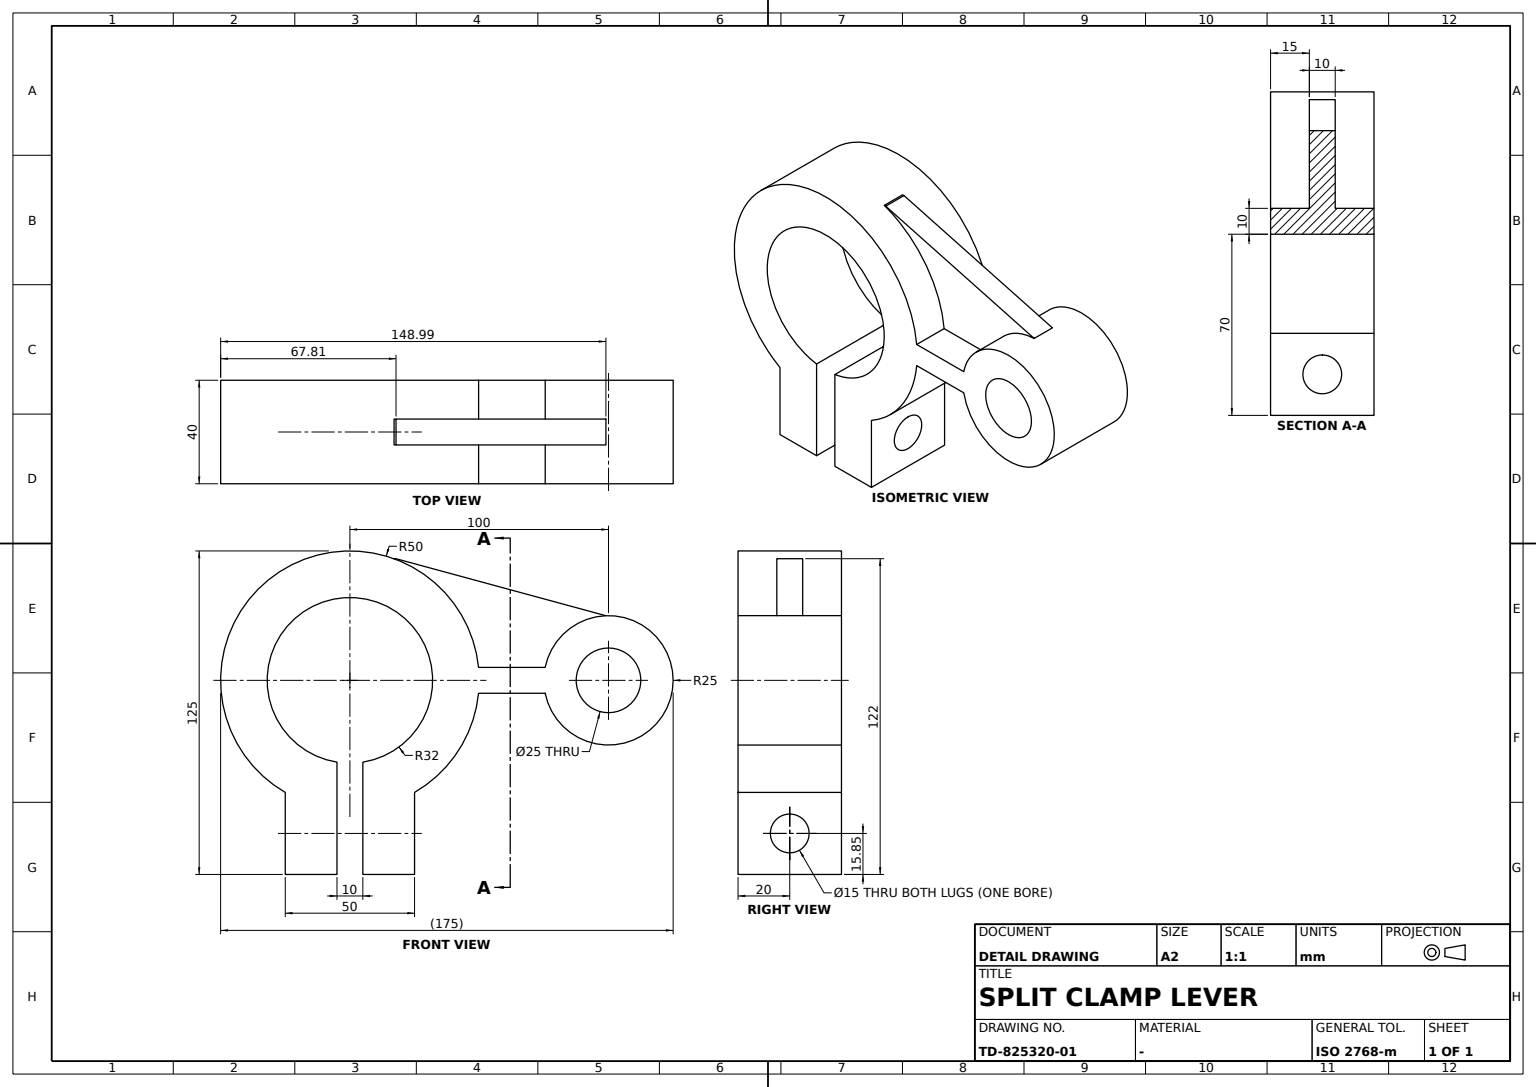
ISO-10303-21;
HEADER;
FILE_DESCRIPTION((''),'2;1');
FILE_NAME('','',(''),(''),'','','');
FILE_SCHEMA(('AUTOMOTIVE_DESIGN'));
ENDSEC;
DATA;
#1=APPLICATION_CONTEXT('');
#2=PRODUCT_CONTEXT('',#1,'mechanical');
#3=PRODUCT('','','',(#2));
#4=PRODUCT_DEFINITION_FORMATION('','',#3);
#5=PRODUCT_DEFINITION_CONTEXT('',#1,'design');
#6=PRODUCT_DEFINITION('','',#4,#5);
#7=PRODUCT_DEFINITION_SHAPE('','',#6);
#8=(LENGTH_UNIT()NAMED_UNIT(*)SI_UNIT(.MILLI.,.METRE.));
#9=(NAMED_UNIT(*)PLANE_ANGLE_UNIT()SI_UNIT($,.RADIAN.));
#10=(NAMED_UNIT(*)SI_UNIT($,.STERADIAN.)SOLID_ANGLE_UNIT());
#11=UNCERTAINTY_MEASURE_WITH_UNIT(LENGTH_MEASURE(0.005),#8,'distance_accuracy_value','');
#12=(GEOMETRIC_REPRESENTATION_CONTEXT(3)GLOBAL_UNCERTAINTY_ASSIGNED_CONTEXT((#11))GLOBAL_UNIT_ASSIGNED_CONTEXT((#8,#9,#10))REPRESENTATION_CONTEXT('',''));
#13=CARTESIAN_POINT('',(5.,116.108107,99.979388));
#14=VERTEX_POINT('',#13);
#15=CARTESIAN_POINT('',(5.,34.936643,122.));
#16=VERTEX_POINT('',#15);
#17=DIRECTION('',(0.,-0.965116262,0.261821696));
#18=VECTOR('',#17,1000.);
#19=LINE('',#13,#18);
#20=EDGE_CURVE('',#14,#16,#19,.T.);
#21=ORIENTED_EDGE('',*,*,#20,.T.);
#22=CARTESIAN_POINT('',(5.,34.181796,122.));
#23=VERTEX_POINT('',#22);
#24=CARTESIAN_POINT('',(5.,129.288452,122.));
#25=DIRECTION('',(0.,-1.,0.));
#26=VECTOR('',#25,1000.);
#27=LINE('',#24,#26);
#28=EDGE_CURVE('',#16,#23,#27,.T.);
#29=ORIENTED_EDGE('',*,*,#28,.T.);
#30=CARTESIAN_POINT('',(5.,66.872445,80.));
#31=VERTEX_POINT('',#30);
#32=CARTESIAN_POINT('',(5.,17.123074,75.));
#33=DIRECTION('',(1.,0.,0.));
#34=DIRECTION('',(0.,0.,-1.));
#35=AXIS2_PLACEMENT_3D('',#32,#33,#34);
#36=CIRCLE('',#35,50.);
#37=EDGE_CURVE('',#31,#23,#36,.T.);
#38=ORIENTED_EDGE('',*,*,#37,.F.);
#39=CARTESIAN_POINT('',(5.,92.628176,80.));
#40=VERTEX_POINT('',#39);
#41=CARTESIAN_POINT('',(5.,129.288452,80.));
#42=DIRECTION('',(0.,1.,0.));
#43=VECTOR('',#42,1000.);
#44=LINE('',#41,#43);
#45=EDGE_CURVE('',#31,#40,#44,.T.);
#46=ORIENTED_EDGE('',*,*,#45,.T.);
#47=CARTESIAN_POINT('',(5.,117.123074,75.));
#48=AXIS2_PLACEMENT_3D('',#47,#33,#34);
#49=CIRCLE('',#48,25.);
#50=EDGE_CURVE('',#14,#40,#49,.T.);
#51=ORIENTED_EDGE('',*,*,#50,.F.);
#52=EDGE_LOOP('',(#21,#29,#38,#46,#51));
#53=FACE_BOUND('',#52,.T.);
#54=CARTESIAN_POINT('',(5.,129.288452,114.));
#55=AXIS2_PLACEMENT_3D('',#54,#33,#25);
#56=PLANE('',#55);
#57=ADVANCED_FACE('',(#53),#56,.T.);
#58=CARTESIAN_POINT('',(-5.,34.181796,122.));
#59=VERTEX_POINT('',#58);
#60=VECTOR('',#33,1000.);
#61=LINE('',#22,#60);
#62=EDGE_CURVE('',#23,#59,#61,.F.);
#63=ORIENTED_EDGE('',*,*,#62,.F.);
#64=ORIENTED_EDGE('',*,*,#28,.F.);
#65=CARTESIAN_POINT('',(-5.,34.936643,122.));
#66=VERTEX_POINT('',#65);
#67=DIRECTION('',(-1.,0.,0.));
#68=VECTOR('',#67,1000.);
#69=LINE('',#15,#68);
#70=EDGE_CURVE('',#16,#66,#69,.T.);
#71=ORIENTED_EDGE('',*,*,#70,.T.);
#72=CARTESIAN_POINT('',(-5.,19.127685,122.));
#73=LINE('',#72,#43);
#74=EDGE_CURVE('',#59,#66,#73,.T.);
#75=ORIENTED_EDGE('',*,*,#74,.F.);
#76=EDGE_LOOP('',(#63,#64,#71,#75));
#77=FACE_BOUND('',#76,.T.);
#78=CARTESIAN_POINT('',(0.,0.,122.));
#79=DIRECTION('',(0.,0.,1.));
#80=AXIS2_PLACEMENT_3D('',#78,#79,#67);
#81=PLANE('',#80);
#82=ADVANCED_FACE('',(#77),#81,.T.);
#83=CARTESIAN_POINT('',(0.,12.123074,8.3495));
#84=VERTEX_POINT('',#83);
#85=CARTESIAN_POINT('',(0.,12.123074,15.8495));
#86=AXIS2_PLACEMENT_3D('',#85,#25,#34);
#87=CIRCLE('',#86,7.5);
#88=EDGE_CURVE('',#84,#84,#87,.T.);
#89=ORIENTED_EDGE('',*,*,#88,.F.);
#90=EDGE_LOOP('',(#89));
#91=FACE_BOUND('',#90,.T.);
#92=CARTESIAN_POINT('',(0.,-7.876926,8.3495));
#93=VERTEX_POINT('',#92);
#94=CARTESIAN_POINT('',(0.,-7.876926,15.8495));
#95=AXIS2_PLACEMENT_3D('',#94,#25,#34);
#96=CIRCLE('',#95,7.5);
#97=EDGE_CURVE('',#93,#93,#96,.T.);
#98=ORIENTED_EDGE('',*,*,#97,.T.);
#99=EDGE_LOOP('',(#98));
#100=FACE_BOUND('',#99,.T.);
#101=CARTESIAN_POINT('',(0.,42.023074,15.8495));
#102=AXIS2_PLACEMENT_3D('',#101,#25,#33);
#103=CYLINDRICAL_SURFACE('',#102,7.5);
#104=ADVANCED_FACE('',(#91,#100),#103,.F.);
#105=CARTESIAN_POINT('',(-20.,22.123074,0.));
#106=VERTEX_POINT('',#105);
#107=CARTESIAN_POINT('',(20.,22.123074,0.));
#108=VERTEX_POINT('',#107);
#109=CARTESIAN_POINT('',(0.,22.123074,0.));
#110=LINE('',#109,#60);
#111=EDGE_CURVE('',#106,#108,#110,.T.);
#112=ORIENTED_EDGE('',*,*,#111,.F.);
#113=CARTESIAN_POINT('',(-20.,42.123074,0.));
#114=VERTEX_POINT('',#113);
#115=CARTESIAN_POINT('',(-20.,0.,0.));
#116=LINE('',#115,#26);
#117=EDGE_CURVE('',#114,#106,#116,.T.);
#118=ORIENTED_EDGE('',*,*,#117,.F.);
#119=CARTESIAN_POINT('',(20.,42.123074,0.));
#120=VERTEX_POINT('',#119);
#121=CARTESIAN_POINT('',(0.,42.123074,0.));
#122=LINE('',#121,#60);
#123=EDGE_CURVE('',#114,#120,#122,.T.);
#124=ORIENTED_EDGE('',*,*,#123,.T.);
#125=CARTESIAN_POINT('',(20.,0.,0.));
#126=LINE('',#125,#26);
#127=EDGE_CURVE('',#120,#108,#126,.T.);
#128=ORIENTED_EDGE('',*,*,#127,.T.);
#129=EDGE_LOOP('',(#112,#118,#124,#128));
#130=FACE_BOUND('',#129,.T.);
#131=CARTESIAN_POINT('',(0.,12.123074,0.));
#132=AXIS2_PLACEMENT_3D('',#131,#79,#25);
#133=PLANE('',#132);
#134=ADVANCED_FACE('',(#130),#133,.F.);
#135=CARTESIAN_POINT('',(-20.,66.872445,80.));
#136=VERTEX_POINT('',#135);
#137=CARTESIAN_POINT('',(-5.,66.872445,80.));
#138=VERTEX_POINT('',#137);
#139=LINE('',#135,#60);
#140=EDGE_CURVE('',#136,#138,#139,.T.);
#141=ORIENTED_EDGE('',*,*,#140,.T.);
#142=CARTESIAN_POINT('',(-5.,92.628176,80.));
#143=VERTEX_POINT('',#142);
#144=LINE('',#137,#43);
#145=EDGE_CURVE('',#138,#143,#144,.T.);
#146=ORIENTED_EDGE('',*,*,#145,.T.);
#147=CARTESIAN_POINT('',(-20.,92.628176,80.));
#148=VERTEX_POINT('',#147);
#149=LINE('',#147,#60);
#150=EDGE_CURVE('',#148,#143,#149,.T.);
#151=ORIENTED_EDGE('',*,*,#150,.F.);
#152=CARTESIAN_POINT('',(-20.,0.,80.));
#153=LINE('',#152,#43);
#154=EDGE_CURVE('',#136,#148,#153,.T.);
#155=ORIENTED_EDGE('',*,*,#154,.F.);
#156=EDGE_LOOP('',(#141,#146,#151,#155));
#157=FACE_BOUND('',#156,.T.);
#158=CARTESIAN_POINT('',(0.,66.872445,80.));
#159=AXIS2_PLACEMENT_3D('',#158,#34,#42);
#160=PLANE('',#159);
#161=ADVANCED_FACE('',(#157),#160,.F.);
#162=CARTESIAN_POINT('',(0.,22.123074,8.3495));
#163=VERTEX_POINT('',#162);
#164=CARTESIAN_POINT('',(0.,22.123074,15.8495));
#165=AXIS2_PLACEMENT_3D('',#164,#25,#34);
#166=CIRCLE('',#165,7.5);
#167=EDGE_CURVE('',#163,#163,#166,.T.);
#168=ORIENTED_EDGE('',*,*,#167,.F.);
#169=EDGE_LOOP('',(#168));
#170=FACE_BOUND('',#169,.T.);
#171=CARTESIAN_POINT('',(-20.,22.123074,43.393039));
#172=VERTEX_POINT('',#171);
#173=VECTOR('',#34,1000.);
#174=LINE('',#105,#173);
#175=EDGE_CURVE('',#172,#106,#174,.T.);
#176=ORIENTED_EDGE('',*,*,#175,.T.);
#177=ORIENTED_EDGE('',*,*,#111,.T.);
#178=CARTESIAN_POINT('',(20.,22.123074,43.393039));
#179=VERTEX_POINT('',#178);
#180=LINE('',#107,#173);
#181=EDGE_CURVE('',#179,#108,#180,.T.);
#182=ORIENTED_EDGE('',*,*,#181,.F.);
#183=LINE('',#171,#60);
#184=EDGE_CURVE('',#172,#179,#183,.T.);
#185=ORIENTED_EDGE('',*,*,#184,.F.);
#186=EDGE_LOOP('',(#176,#177,#182,#185));
#187=FACE_BOUND('',#186,.T.);
#188=CARTESIAN_POINT('',(0.,22.123074,43.393039));
#189=AXIS2_PLACEMENT_3D('',#188,#25,#34);
#190=PLANE('',#189);
#191=ADVANCED_FACE('',(#170,#187),#190,.T.);
#192=CARTESIAN_POINT('',(20.,42.123074,31.69873));
#193=VERTEX_POINT('',#192);
#194=CARTESIAN_POINT('',(20.,66.872445,70.));
#195=VERTEX_POINT('',#194);
#196=CARTESIAN_POINT('',(20.,17.123074,75.));
#197=AXIS2_PLACEMENT_3D('',#196,#33,#34);
#198=CIRCLE('',#197,50.);
#199=EDGE_CURVE('',#193,#195,#198,.T.);
#200=ORIENTED_EDGE('',*,*,#199,.F.);
#201=CARTESIAN_POINT('',(-20.,42.123074,31.69873));
#202=VERTEX_POINT('',#201);
#203=LINE('',#201,#60);
#204=EDGE_CURVE('',#202,#193,#203,.T.);
#205=ORIENTED_EDGE('',*,*,#204,.F.);
#206=CARTESIAN_POINT('',(-20.,66.872445,70.));
#207=VERTEX_POINT('',#206);
#208=CARTESIAN_POINT('',(-20.,17.123074,75.));
#209=AXIS2_PLACEMENT_3D('',#208,#33,#34);
#210=CIRCLE('',#209,50.);
#211=EDGE_CURVE('',#202,#207,#210,.T.);
#212=ORIENTED_EDGE('',*,*,#211,.T.);
#213=LINE('',#206,#60);
#214=EDGE_CURVE('',#207,#195,#213,.T.);
#215=ORIENTED_EDGE('',*,*,#214,.T.);
#216=EDGE_LOOP('',(#200,#205,#212,#215));
#217=FACE_BOUND('',#216,.T.);
#218=CARTESIAN_POINT('',(0.,17.123074,75.));
#219=AXIS2_PLACEMENT_3D('',#218,#33,#42);
#220=CYLINDRICAL_SURFACE('',#219,50.);
#221=ADVANCED_FACE('',(#217),#220,.T.);
#222=ORIENTED_EDGE('',*,*,#97,.F.);
#223=EDGE_LOOP('',(#222));
#224=FACE_BOUND('',#223,.T.);
#225=CARTESIAN_POINT('',(-20.,-7.876926,0.));
#226=VERTEX_POINT('',#225);
#227=CARTESIAN_POINT('',(20.,-7.876926,0.));
#228=VERTEX_POINT('',#227);
#229=CARTESIAN_POINT('',(0.,-7.876926,0.));
#230=LINE('',#229,#60);
#231=EDGE_CURVE('',#226,#228,#230,.T.);
#232=ORIENTED_EDGE('',*,*,#231,.T.);
#233=CARTESIAN_POINT('',(20.,-7.876926,31.69873));
#234=VERTEX_POINT('',#233);
#235=LINE('',#227,#173);
#236=EDGE_CURVE('',#234,#228,#235,.T.);
#237=ORIENTED_EDGE('',*,*,#236,.F.);
#238=CARTESIAN_POINT('',(-20.,-7.876926,31.69873));
#239=VERTEX_POINT('',#238);
#240=LINE('',#238,#60);
#241=EDGE_CURVE('',#239,#234,#240,.T.);
#242=ORIENTED_EDGE('',*,*,#241,.F.);
#243=LINE('',#225,#173);
#244=EDGE_CURVE('',#239,#226,#243,.T.);
#245=ORIENTED_EDGE('',*,*,#244,.T.);
#246=EDGE_LOOP('',(#232,#237,#242,#245));
#247=FACE_BOUND('',#246,.T.);
#248=CARTESIAN_POINT('',(0.,-7.876926,31.69873));
#249=AXIS2_PLACEMENT_3D('',#248,#25,#34);
#250=PLANE('',#249);
#251=ADVANCED_FACE('',(#224,#247),#250,.T.);
#252=ORIENTED_EDGE('',*,*,#167,.T.);
#253=EDGE_LOOP('',(#252));
#254=FACE_BOUND('',#253,.T.);
#255=CARTESIAN_POINT('',(0.,42.123074,23.3495));
#256=VERTEX_POINT('',#255);
#257=CARTESIAN_POINT('',(0.,42.123074,15.8495));
#258=AXIS2_PLACEMENT_3D('',#257,#42,#79);
#259=CIRCLE('',#258,7.5);
#260=EDGE_CURVE('',#256,#256,#259,.T.);
#261=ORIENTED_EDGE('',*,*,#260,.T.);
#262=EDGE_LOOP('',(#261));
#263=FACE_BOUND('',#262,.T.);
#264=ADVANCED_FACE('',(#254,#263),#103,.F.);
#265=CARTESIAN_POINT('',(-20.,12.123074,0.));
#266=VERTEX_POINT('',#265);
#267=CARTESIAN_POINT('',(20.,12.123074,0.));
#268=VERTEX_POINT('',#267);
#269=LINE('',#131,#60);
#270=EDGE_CURVE('',#266,#268,#269,.T.);
#271=ORIENTED_EDGE('',*,*,#270,.T.);
#272=EDGE_CURVE('',#268,#228,#126,.T.);
#273=ORIENTED_EDGE('',*,*,#272,.T.);
#274=ORIENTED_EDGE('',*,*,#231,.F.);
#275=EDGE_CURVE('',#266,#226,#116,.T.);
#276=ORIENTED_EDGE('',*,*,#275,.F.);
#277=EDGE_LOOP('',(#271,#273,#274,#276));
#278=FACE_BOUND('',#277,.T.);
#279=ADVANCED_FACE('',(#278),#133,.F.);
#280=CARTESIAN_POINT('',(-20.,92.628176,70.));
#281=VERTEX_POINT('',#280);
#282=CARTESIAN_POINT('',(20.,92.628176,70.));
#283=VERTEX_POINT('',#282);
#284=LINE('',#280,#60);
#285=EDGE_CURVE('',#281,#283,#284,.T.);
#286=ORIENTED_EDGE('',*,*,#285,.T.);
#287=CARTESIAN_POINT('',(20.,0.,70.));
#288=LINE('',#287,#26);
#289=EDGE_CURVE('',#283,#195,#288,.T.);
#290=ORIENTED_EDGE('',*,*,#289,.T.);
#291=ORIENTED_EDGE('',*,*,#214,.F.);
#292=CARTESIAN_POINT('',(-20.,0.,70.));
#293=LINE('',#292,#26);
#294=EDGE_CURVE('',#281,#207,#293,.T.);
#295=ORIENTED_EDGE('',*,*,#294,.F.);
#296=EDGE_LOOP('',(#286,#290,#291,#295));
#297=FACE_BOUND('',#296,.T.);
#298=CARTESIAN_POINT('',(0.,92.628176,70.));
#299=AXIS2_PLACEMENT_3D('',#298,#79,#25);
#300=PLANE('',#299);
#301=ADVANCED_FACE('',(#297),#300,.F.);
#302=ORIENTED_EDGE('',*,*,#184,.T.);
#303=CARTESIAN_POINT('',(20.,12.123074,43.393039));
#304=VERTEX_POINT('',#303);
#305=CIRCLE('',#197,32.);
#306=EDGE_CURVE('',#179,#304,#305,.T.);
#307=ORIENTED_EDGE('',*,*,#306,.T.);
#308=CARTESIAN_POINT('',(-20.,12.123074,43.393039));
#309=VERTEX_POINT('',#308);
#310=LINE('',#308,#60);
#311=EDGE_CURVE('',#309,#304,#310,.T.);
#312=ORIENTED_EDGE('',*,*,#311,.F.);
#313=CIRCLE('',#209,32.);
#314=EDGE_CURVE('',#172,#309,#313,.T.);
#315=ORIENTED_EDGE('',*,*,#314,.F.);
#316=EDGE_LOOP('',(#302,#307,#312,#315));
#317=FACE_BOUND('',#316,.T.);
#318=CYLINDRICAL_SURFACE('',#219,32.);
#319=ADVANCED_FACE('',(#317),#318,.F.);
#320=CARTESIAN_POINT('',(-20.,117.123074,62.5));
#321=VERTEX_POINT('',#320);
#322=CARTESIAN_POINT('',(-20.,117.123074,75.));
#323=AXIS2_PLACEMENT_3D('',#322,#33,#34);
#324=CIRCLE('',#323,12.5);
#325=EDGE_CURVE('',#321,#321,#324,.T.);
#326=ORIENTED_EDGE('',*,*,#325,.F.);
#327=EDGE_LOOP('',(#326));
#328=FACE_BOUND('',#327,.T.);
#329=CARTESIAN_POINT('',(20.,117.123074,62.5));
#330=VERTEX_POINT('',#329);
#331=CARTESIAN_POINT('',(20.,117.123074,75.));
#332=AXIS2_PLACEMENT_3D('',#331,#33,#34);
#333=CIRCLE('',#332,12.5);
#334=EDGE_CURVE('',#330,#330,#333,.T.);
#335=ORIENTED_EDGE('',*,*,#334,.T.);
#336=EDGE_LOOP('',(#335));
#337=FACE_BOUND('',#336,.T.);
#338=CARTESIAN_POINT('',(19.9,117.123074,75.));
#339=AXIS2_PLACEMENT_3D('',#338,#67,#42);
#340=CYLINDRICAL_SURFACE('',#339,12.5);
#341=ADVANCED_FACE('',(#328,#337),#340,.F.);
#342=ORIENTED_EDGE('',*,*,#325,.T.);
#343=EDGE_LOOP('',(#342));
#344=FACE_BOUND('',#343,.T.);
#345=ORIENTED_EDGE('',*,*,#314,.T.);
#346=LINE('',#265,#173);
#347=EDGE_CURVE('',#309,#266,#346,.T.);
#348=ORIENTED_EDGE('',*,*,#347,.T.);
#349=ORIENTED_EDGE('',*,*,#275,.T.);
#350=ORIENTED_EDGE('',*,*,#244,.F.);
#351=EDGE_CURVE('',#136,#239,#210,.T.);
#352=ORIENTED_EDGE('',*,*,#351,.F.);
#353=ORIENTED_EDGE('',*,*,#154,.T.);
#354=CIRCLE('',#323,25.);
#355=EDGE_CURVE('',#281,#148,#354,.T.);
#356=ORIENTED_EDGE('',*,*,#355,.F.);
#357=ORIENTED_EDGE('',*,*,#294,.T.);
#358=ORIENTED_EDGE('',*,*,#211,.F.);
#359=VECTOR('',#79,1000.);
#360=LINE('',#113,#359);
#361=EDGE_CURVE('',#114,#202,#360,.T.);
#362=ORIENTED_EDGE('',*,*,#361,.F.);
#363=ORIENTED_EDGE('',*,*,#117,.T.);
#364=ORIENTED_EDGE('',*,*,#175,.F.);
#365=EDGE_LOOP('',(#345,#348,#349,#350,#352,#353,#356,#357,#358,#362,#363,#364));
#366=FACE_BOUND('',#365,.T.);
#367=AXIS2_PLACEMENT_3D('',#115,#33,#42);
#368=PLANE('',#367);
#369=ADVANCED_FACE('',(#344,#366),#368,.F.);
#370=CARTESIAN_POINT('',(-5.,116.108107,99.979388));
#371=VERTEX_POINT('',#370);
#372=LINE('',#13,#60);
#373=EDGE_CURVE('',#14,#371,#372,.F.);
#374=ORIENTED_EDGE('',*,*,#373,.F.);
#375=ORIENTED_EDGE('',*,*,#50,.T.);
#376=CARTESIAN_POINT('',(20.,92.628176,80.));
#377=VERTEX_POINT('',#376);
#378=LINE('',#39,#60);
#379=EDGE_CURVE('',#40,#377,#378,.T.);
#380=ORIENTED_EDGE('',*,*,#379,.T.);
#381=CIRCLE('',#332,25.);
#382=EDGE_CURVE('',#283,#377,#381,.T.);
#383=ORIENTED_EDGE('',*,*,#382,.F.);
#384=ORIENTED_EDGE('',*,*,#285,.F.);
#385=ORIENTED_EDGE('',*,*,#355,.T.);
#386=ORIENTED_EDGE('',*,*,#150,.T.);
#387=CARTESIAN_POINT('',(-5.,117.123074,75.));
#388=AXIS2_PLACEMENT_3D('',#387,#67,#79);
#389=CIRCLE('',#388,25.);
#390=EDGE_CURVE('',#143,#371,#389,.T.);
#391=ORIENTED_EDGE('',*,*,#390,.T.);
#392=EDGE_LOOP('',(#374,#375,#380,#383,#384,#385,#386,#391));
#393=FACE_BOUND('',#392,.T.);
#394=CARTESIAN_POINT('',(-12.5,117.123074,75.));
#395=AXIS2_PLACEMENT_3D('',#394,#33,#42);
#396=CYLINDRICAL_SURFACE('',#395,25.);
#397=ADVANCED_FACE('',(#393),#396,.T.);
#398=ORIENTED_EDGE('',*,*,#88,.T.);
#399=EDGE_LOOP('',(#398));
#400=FACE_BOUND('',#399,.T.);
#401=ORIENTED_EDGE('',*,*,#347,.F.);
#402=ORIENTED_EDGE('',*,*,#311,.T.);
#403=LINE('',#267,#173);
#404=EDGE_CURVE('',#304,#268,#403,.T.);
#405=ORIENTED_EDGE('',*,*,#404,.T.);
#406=ORIENTED_EDGE('',*,*,#270,.F.);
#407=EDGE_LOOP('',(#401,#402,#405,#406));
#408=FACE_BOUND('',#407,.T.);
#409=CARTESIAN_POINT('',(0.,12.123074,43.393039));
#410=AXIS2_PLACEMENT_3D('',#409,#25,#34);
#411=PLANE('',#410);
#412=ADVANCED_FACE('',(#400,#408),#411,.F.);
#413=ORIENTED_EDGE('',*,*,#62,.T.);
#414=CARTESIAN_POINT('',(-5.,17.123074,75.));
#415=AXIS2_PLACEMENT_3D('',#414,#67,#79);
#416=CIRCLE('',#415,50.);
#417=EDGE_CURVE('',#59,#138,#416,.T.);
#418=ORIENTED_EDGE('',*,*,#417,.T.);
#419=ORIENTED_EDGE('',*,*,#140,.F.);
#420=ORIENTED_EDGE('',*,*,#351,.T.);
#421=ORIENTED_EDGE('',*,*,#241,.T.);
#422=CARTESIAN_POINT('',(20.,66.872445,80.));
#423=VERTEX_POINT('',#422);
#424=EDGE_CURVE('',#423,#234,#198,.T.);
#425=ORIENTED_EDGE('',*,*,#424,.F.);
#426=LINE('',#30,#60);
#427=EDGE_CURVE('',#31,#423,#426,.T.);
#428=ORIENTED_EDGE('',*,*,#427,.F.);
#429=ORIENTED_EDGE('',*,*,#37,.T.);
#430=EDGE_LOOP('',(#413,#418,#419,#420,#421,#425,#428,#429));
#431=FACE_BOUND('',#430,.T.);
#432=ADVANCED_FACE('',(#431),#220,.T.);
#433=ORIENTED_EDGE('',*,*,#260,.F.);
#434=EDGE_LOOP('',(#433));
#435=FACE_BOUND('',#434,.T.);
#436=LINE('',#119,#359);
#437=EDGE_CURVE('',#120,#193,#436,.T.);
#438=ORIENTED_EDGE('',*,*,#437,.F.);
#439=ORIENTED_EDGE('',*,*,#123,.F.);
#440=ORIENTED_EDGE('',*,*,#361,.T.);
#441=ORIENTED_EDGE('',*,*,#204,.T.);
#442=EDGE_LOOP('',(#438,#439,#440,#441));
#443=FACE_BOUND('',#442,.T.);
#444=AXIS2_PLACEMENT_3D('',#121,#42,#79);
#445=PLANE('',#444);
#446=ADVANCED_FACE('',(#435,#443),#445,.T.);
#447=ORIENTED_EDGE('',*,*,#70,.F.);
#448=ORIENTED_EDGE('',*,*,#20,.F.);
#449=ORIENTED_EDGE('',*,*,#373,.T.);
#450=DIRECTION('',(0.,0.965116262,-0.261821696));
#451=VECTOR('',#450,1000.);
#452=LINE('',#370,#451);
#453=EDGE_CURVE('',#66,#371,#452,.T.);
#454=ORIENTED_EDGE('',*,*,#453,.F.);
#455=EDGE_LOOP('',(#447,#448,#449,#454));
#456=FACE_BOUND('',#455,.T.);
#457=DIRECTION('',(0.,-0.261821696,-0.965116262));
#458=AXIS2_PLACEMENT_3D('',#13,#457,#17);
#459=PLANE('',#458);
#460=ADVANCED_FACE('',(#456),#459,.F.);
#461=ORIENTED_EDGE('',*,*,#74,.T.);
#462=ORIENTED_EDGE('',*,*,#453,.T.);
#463=ORIENTED_EDGE('',*,*,#390,.F.);
#464=ORIENTED_EDGE('',*,*,#145,.F.);
#465=ORIENTED_EDGE('',*,*,#417,.F.);
#466=EDGE_LOOP('',(#461,#462,#463,#464,#465));
#467=FACE_BOUND('',#466,.T.);
#468=CARTESIAN_POINT('',(-5.,19.127685,114.));
#469=AXIS2_PLACEMENT_3D('',#468,#67,#42);
#470=PLANE('',#469);
#471=ADVANCED_FACE('',(#467),#470,.T.);
#472=ORIENTED_EDGE('',*,*,#427,.T.);
#473=CARTESIAN_POINT('',(20.,0.,80.));
#474=LINE('',#473,#43);
#475=EDGE_CURVE('',#423,#377,#474,.T.);
#476=ORIENTED_EDGE('',*,*,#475,.T.);
#477=ORIENTED_EDGE('',*,*,#379,.F.);
#478=ORIENTED_EDGE('',*,*,#45,.F.);
#479=EDGE_LOOP('',(#472,#476,#477,#478));
#480=FACE_BOUND('',#479,.T.);
#481=ADVANCED_FACE('',(#480),#160,.F.);
#482=ORIENTED_EDGE('',*,*,#272,.F.);
#483=ORIENTED_EDGE('',*,*,#404,.F.);
#484=ORIENTED_EDGE('',*,*,#306,.F.);
#485=ORIENTED_EDGE('',*,*,#181,.T.);
#486=ORIENTED_EDGE('',*,*,#127,.F.);
#487=ORIENTED_EDGE('',*,*,#437,.T.);
#488=ORIENTED_EDGE('',*,*,#199,.T.);
#489=ORIENTED_EDGE('',*,*,#289,.F.);
#490=ORIENTED_EDGE('',*,*,#382,.T.);
#491=ORIENTED_EDGE('',*,*,#475,.F.);
#492=ORIENTED_EDGE('',*,*,#424,.T.);
#493=ORIENTED_EDGE('',*,*,#236,.T.);
#494=EDGE_LOOP('',(#482,#483,#484,#485,#486,#487,#488,#489,#490,#491,#492,#493));
#495=FACE_BOUND('',#494,.T.);
#496=ORIENTED_EDGE('',*,*,#334,.F.);
#497=EDGE_LOOP('',(#496));
#498=FACE_BOUND('',#497,.T.);
#499=AXIS2_PLACEMENT_3D('',#125,#33,#42);
#500=PLANE('',#499);
#501=ADVANCED_FACE('',(#495,#498),#500,.T.);
#502=CLOSED_SHELL('',(#57,#82,#104,#134,#161,#191,#221,#251,#264,#279,#301,#319,#341,#369,#397,#412,#432,#446,#460,#471,#481,#501));
#503=MANIFOLD_SOLID_BREP('',#502);
#504=ADVANCED_BREP_SHAPE_REPRESENTATION('',(#503),#12);
#505=SHAPE_DEFINITION_REPRESENTATION(#7,#504);
ENDSEC;
END-ISO-10303-21;
